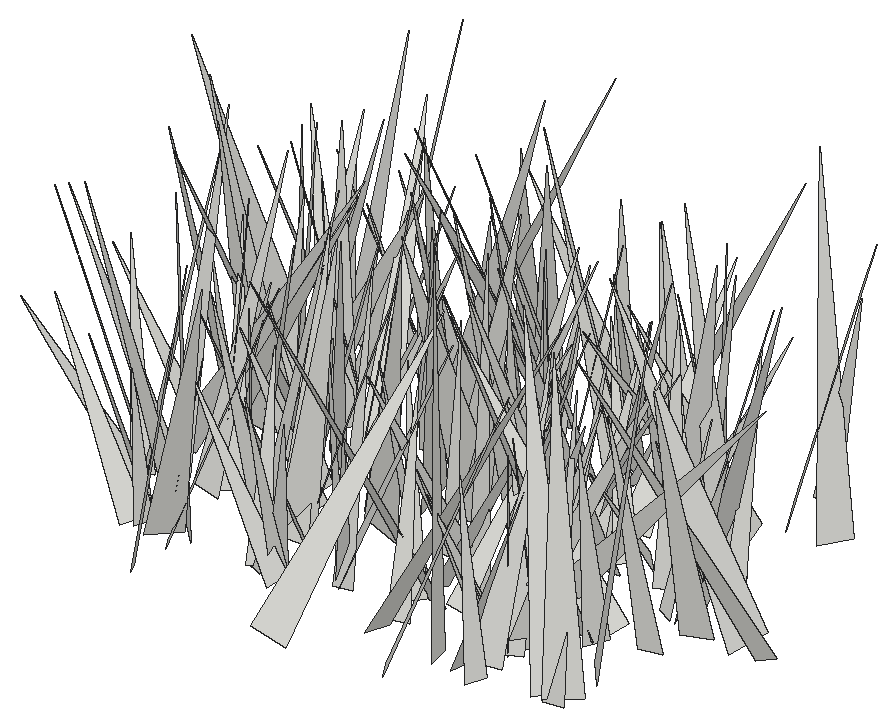
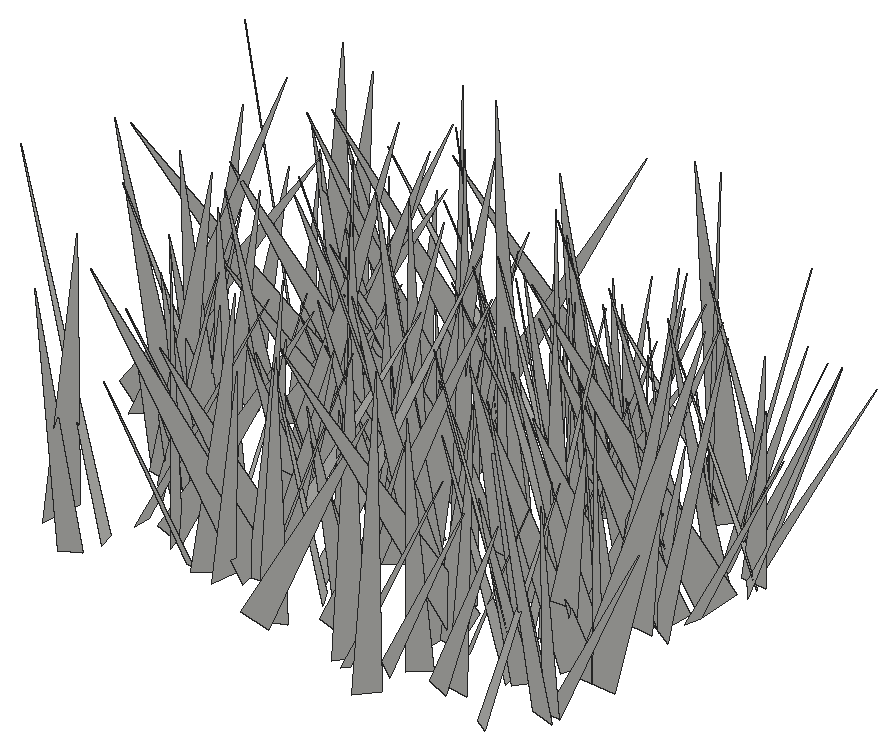
# SketchUp Ruby script. Lengths in inches.
U = 1.inch
M = Sketchup.active_model
def pt(a) = Geom::Point3d.new(a.map { |v| v * U })
def face(e, loops, mat)
  f = e.add_face(loops[0].map { |a| pt(a) })
  loops[1..].each { |l| e.add_face(l.map { |a| pt(a) }).erase! }
  f.material = f.back_material = mat if mat
  f
end
# faces: each face lists its corners as indices into pts; further lists are holes
def faces(e, pts, list, mat = nil) = list.each { |f| face(e, (f[0].is_a?(Array) ? f : [f]).map { |l| l.map { |i| pts[i] } }, mat) }
# xy, xz, yz: faces in a plane at the given z, y or x. An outline is a flat list of corners, or four numbers for a rectangle; further outlines are holes
def ring(l) = l.size == 4 ? [[l[0], l[1]], [l[2], l[1]], [l[2], l[3]], [l[0], l[3]]] : l.each_slice(2).to_a
def flat(e, list, mat, &to3) = list.each { |f| face(e, (f[0].is_a?(Array) ? f : [f]).map { |l| ring(l).map { |u, v| to3.(u, v) } }, mat) }
def xy(e, z, list, mat = nil) = flat(e, list, mat) { |x, y| [x, y, z] }
def xz(e, y, list, mat = nil) = flat(e, list, mat) { |x, z| [x, y, z] }
def yz(e, x, list, mat = nil) = flat(e, list, mat) { |y, z| [x, y, z] }
def lines(e, pts, list) = list.each { |a, b| e.add_line(pt(pts[a]), pt(pts[b])) }
# prism: a flat outline (further loops are holes) pulled along v
def prism(e, loops, v, mat = nil)
  f = face(e, loops, mat); d = Geom::Vector3d.new(v.map { |x| x * U })
  f.pushpull(f.normal.samedirection?(d) ? d.length : -d.length)
end
def box(e, o, s, mat = nil) = prism(e, [[o, [o[0] + s[0], o[1], o[2]], [o[0] + s[0], o[1] + s[1], o[2]], [o[0], o[1] + s[1], o[2]]]], [0, 0, s[2]], mat)
def at(x, y, z, deg = 0) = Geom::Transformation.translation(pt([x, y, z])) * Geom::Transformation.rotation(ORIGIN, Z_AXIS, deg.degrees)
def axes(o, x, y, z) = Geom::Transformation.new([*x, 0, *y, 0, *z, 0, *pt(o).to_a, 1])
def part(name) = M.definitions.add(name)
# library, detail: a bought-in or finely detailed component or shape, given as its bounding box
def library(name, o, s) = part(name).tap { |d| box(d.entities, o, s) }
def detail(e, o, s) = box(e.add_group.entities, o, s)
def put(e, d, t, mat = nil) = e.add_instance(d, t).tap { |i| i.material = mat if mat }
def group(e, t, mat = nil) = e.add_group.tap { |g| g.transformation = t; g.material = mat if mat }.entities
root = M.entities
c1 = part("fur_instance\#9")
p = [[0.8125,0,1.79],[0.67,-0.02,1.48],[0,-0.11,0],[0,0.11,0]]
faces(c1.entities,p,[[0,1,2,3]])
put(root,c1,axes([84.93,28.2,-27.1],[-3.91308,1.33626,1.31278],[1.41439,4.10109,0.04154],[1.2282,-0.46546,4.13474]))
put(root,c1,axes([68.6,29.75,-27.1],[5.57249,-4.36069,0.56036],[-4.38496,-5.5781,0.19774],[-0.31889,0.50141,7.07313]))
put(root,c1,axes([81.72,26.67,-27.1],[5.03516,3.5658,0.22039],[3.50469,-5.00395,0.89105],[-0.69327,0.6016,6.10523]))
put(root,c1,axes([76.67,25.97,-27.1],[-0.73588,7.38124,0.25307],[6.98236,0.77818,-2.39362],[2.40696,-0.00075,7.02103]))
put(root,c1,axes([69.36,26.85,-27.1],[4.53649,3.63122,1.57008],[3.09166,-4.74451,2.04009],[-2.46831,0.73111,5.44092]))
put(root,c1,axes([74.26,29.53,-27.1],[-4.45422,0.97791,0.2811],[1.01486,4.3608,0.91044],[0.07343,-0.95002,4.4685]))
put(root,c1,axes([73.88,30.16,-27.1],[-3.9744,-0.24759,1.6573],[0.13335,4.20562,0.94807],[1.67038,-0.92483,3.8676]))
put(root,c1,axes([67.49,29.9,-27.1],[2.92591,-1.89098,1.19539],[-1.88086,-3.14489,-0.37117],[-1.21125,0.31559,3.46396]))
put(root,c1,axes([73.47,30.54,-27.1],[0.57309,-4.07864,0.58369],[-4.03575,-0.43699,0.90892],[0.82985,0.69149,4.01716]))
put(root,c1,axes([67.57,30.38,-27.1],[-2.05359,-3.75931,0.63579],[-3.81243,2.01617,-0.39286],[-0.04503,0.74602,4.26559]))
put(root,c1,axes([88.39,29.16,-27.1],[-4.52139,5.22079,2.42729],[5.56937,4.74843,0.161],[1.45961,-1.94607,6.90462]))
put(root,c1,axes([67.04,29.79,-27.1],[-3.88022,2.75048,0.41463],[2.75578,3.70465,1.21426],[-0.37781,-1.22622,4.59857]))
put(root,c1,axes([69.24,30.39,-27.1],[-4.9247,-5.05159,2.9073],[-5.39927,5.38751,0.21521],[2.19519,1.91829,7.05159]))
put(root,c1,axes([80.1,31.94,-27.1],[-3.80092,-6.72254,0.0507],[-6.48684,3.65215,-2.05545],[-1.76524,1.05421,7.4441]))
put(root,c1,axes([82.68,28.74,-27.1],[-7.45834,-2.27512,2.73301],[-2.96816,7.48025,-1.87304],[1.95846,2.67246,7.56933]))
put(root,c1,axes([84.33,30.9375,-27.1],[-3.42009,-2.62307,1.97794],[-2.56254,3.91671,0.76324],[2.05575,0.51835,4.24205]))
put(root,c1,axes([87.82,29.27,-27.1],[-6.04844,4.67756,1.28768],[4.75602,6.12308,0.0974],[0.95811,-0.86582,7.6455]))
put(root,c1,axes([75.96,31.41,-27.1],[3.91592,-0.46866,0.80636],[-0.26131,-3.89224,-0.99321],[-0.89531,-0.91384,3.81675]))
put(root,c1,axes([84.44,29.37,-27.1],[-2.07384,5.25709,1.74566],[5.26815,2.4479,-1.11335],[1.712,-1.16445,5.54061]))
put(root,c1,axes([88.37,28.6,-27.1],[1.19098,5.93826,0.851],[5.76454,-1.37303,1.51343],[-1.66049,-0.50738,5.86438]))
put(root,c1,axes([82.39,32.1,-27.1],[-3.37943,-0.96857,0.84627],[-0.6019,3.29348,1.36586],[1.13667,-1.13567,3.23931]))
put(root,c1,axes([73,29.98,-27.1],[-1.62337,4.08317,1.17277],[4.21606,1.70273,-0.09236],[0.52201,-1.05424,4.39307]))
put(root,c1,axes([82.14,32.07,-27.1],[0.37183,-3.94608,0.38846],[-3.8933,-0.43727,-0.71534],[-0.75144,0.31297,3.89847]))
put(root,c1,axes([65.42,32.36,-27.1],[-4.70731,-0.314,0.0439],[-0.28456,4.4722,1.47573],[0.13983,-1.46975,4.48103]))
put(root,c1,axes([79.5,29.03,-27.1],[7.73901,0.54751,0.09462],[0.50511,-7.48314,1.98706],[-0.23147,1.9758,7.49957]))
put(root,c1,axes([83.77,28.63,-27.1],[6.82922,2.21825,1.16198],[1.82522,-6.72015,2.10172],[-1.71447,1.68168,6.86597]))
put(root,c1,axes([79.75,29.98,-27.1],[-0.43977,4.5707,0.64422],[4.59918,0.3789,0.45132],[-0.39225,-0.6818,4.56957]))
put(root,c1,axes([69.25,29.11,-27.1],[4.51704,3.2359,0.24642],[3.07452,-4.40221,1.45028],[-1.0388,1.04161,5.3639]))
put(root,c1,axes([66.73,32.49,-27.1],[-6.28754,-2.52373,1.27093],[-2.51372,6.41179,0.29625],[1.29062,0.19325,6.76865]))
put(root,c1,axes([75.96,31.16,-27.1],[4.98455,3.49636,0.32674],[3.50629,-4.92427,-0.79656],[0.19289,-0.83908,6.03621]))
put(root,c1,axes([88.13,31.47,-27.1],[5.88152,4.86813,2.28116],[5.13014,-6.09312,-0.22398],[-1.60749,-1.63397,7.63157]))
put(root,c1,axes([71.04,32.7,-27.1],[-4.89796,-0.50596,1.28828],[-0.38248,5.0478,0.52832],[1.33018,-0.4116,4.8956]))
put(root,c1,axes([66.65,32.99,-27.1],[3.46775,1.51161,0.84573],[1.722,-3.21287,-1.3182],[-0.18693,-1.55498,3.54578]))
put(root,c1,axes([72.72,32.56,-27.1],[2.84119,-6.18581,2.36185],[-6.62137,-2.65127,1.02137],[0.00779,2.57322,6.73004]))
put(root,c1,axes([75.22,32.19,-27.1],[1.82668,3.73793,1.95155],[3.99067,-2.21946,0.51574],[-1.36206,-1.48974,4.1283]))
put(root,c1,axes([84.125,32.78,-27.1],[-3.08736,-2.6391,1.38175],[-2.74426,3.29386,0.15946],[1.15895,0.7691,4.05847]))
put(root,c1,axes([72.91,29.76,-27.1],[4.10406,6.33899,0.98584],[6.11766,-4.2195,1.66374],[-1.93105,0.10466,7.36601]))
put(root,c1,axes([73.32,32.36,-27.1],[-3.16767,-3.69393,0.44061],[-3.42422,2.66901,-2.24153],[-1.45395,1.76199,4.31912]))
put(root,c1,axes([86.07,33.41,-27.1],[-4.08084,-6.31933,0.93728],[-6.28934,3.77891,-1.90517],[-1.12095,1.80323,7.27719]))
put(root,c1,axes([78.36,33.12,-27.1],[-4.55771,-1.35516,1.4154],[-1.26006,4.77117,0.51063],[1.50069,-0.10962,4.72742]))
put(root,c1,axes([79.8125,34.55,-27.1],[1.26749,-5.25605,0.55346],[-5.00773,-1.37633,-1.60227],[-1.68968,0.13629,5.16385]))
put(root,c1,axes([84.64,31.13,-27.1],[4.97283,-0.90694,1.68915],[-1.45035,-4.85051,1.66547],[-1.25389,2.01364,4.77261]))
put(root,c1,axes([86.66,33.32,-27.1],[3.6689,-2.8215,1.45683],[-2.81207,-3.92099,-0.512],[-1.47496,0.45716,4.59995]))
put(root,c1,axes([78.65,31.16,-27.1],[5.2038,5.70361,2.35891],[5.67233,-5.63566,1.11317],[-2.43315,-0.93989,7.64013]))
put(root,c1,axes([82.17,34.89,-27.1],[1.01842,-6.5564,0.3467],[-5.92672,-0.76709,2.90332],[2.82498,0.75429,5.9661]))
put(root,c1,axes([74.91,35,-27.1],[-0.13317,-8.12567,1.45261],[-7.87911,0.55826,2.40046],[2.46092,1.34765,7.76415]))
put(root,c1,axes([76.51,30.67,-27.1],[1.43264,6.02249,0.66756],[5.77311,-1.565,1.72927],[-1.84042,-0.22107,5.94411]))
put(root,c1,axes([79.24,31.66,-27.1],[-4.35702,1.54483,0.37411],[1.45493,4.3157,-0.87633],[0.64002,0.7059,4.53896]))
put(root,c1,axes([84.7,30.58,-27.1],[-5.37291,2.30629,0.61766],[1.96946,5.14098,-2.06404],[1.34972,1.6793,5.47055]))
put(root,c1,axes([65.08,33.22,-27.1],[-4.61833,-3.74237,0.73758],[-3.79853,4.40694,-1.4242],[-0.34716,1.56584,5.77113]))
put(root,c1,axes([84.61,33.04,-27.1],[2.40837,2.51325,1.53163],[2.71206,-2.66382,0.10655],[-1.14326,-1.0248,3.47927]))
put(root,c1,axes([72.71,32.33,-27.1],[-0.45657,6.34549,1.8425],[6.59681,0.54314,-0.23589],[0.37708,-1.81886,6.35752]))
put(root,c1,axes([66.14,33.47,-27.1],[-6.00367,-1.40851,0.07652],[-1.40991,5.98159,-0.51624],[-0.04369,0.52005,6.14503]))
put(root,c1,axes([71.98,34.82,-27.1],[-4.35378,0.44066,1.23045],[0.84047,4.2213,1.46212],[1.0009,-1.62788,4.12453]))
put(root,c1,axes([69.75,33.64,-27.1],[3.22406,2.21993,1.84513],[2.48282,-3.54361,-0.0749],[-1.47248,-1.11442,3.91371]))
put(root,c1,axes([88.67,34.09,-27.1],[-0.10037,-5.00985,1.67679],[-5.24561,-0.10471,-0.62683],[-0.62754,1.67652,4.9715]))
put(root,c1,axes([86.66,34.27,-27.1],[-6.39943,2.86094,0.01202],[2.71801,6.07041,2.2137],[-0.89308,-2.0256,6.65111]))
put(root,c1,axes([83.79,31.79,-27.1],[5.89458,-2.32049,1.52507],[-2.76984,-5.16651,2.8446],[-0.1962,3.22166,5.6603]))
put(root,c1,axes([65.08,32.84,-27.1],[-0.91318,4.58049,0.90258],[4.61205,0.74242,0.89849],[-0.72428,-1.04754,4.5834]))
put(root,c1,axes([80.95,32.06,-27.1],[-0.63847,4.33122,0.11328],[4.14955,0.64421,-1.24344],[1.2464,0.07394,4.19773]))
put(root,c1,axes([83.72,32.78,-27.1],[6.0984,-4.54505,0.22334],[-3.82324,-4.91501,4.37303],[2.46783,3.61705,6.22291]))
put(root,c1,axes([82.7,34.5,-27.1],[-2.40754,3.72637,1.88833],[4.14407,2.40561,0.53634],[0.52762,-1.89079,4.40391]))
put(root,c1,axes([79.36,32.97,-27.1],[5.44463,0.12063,0.24069],[0.04962,-5.23956,1.50366],[-0.26462,1.49964,5.23426]))
put(root,c1,axes([89.36,36.04,-27.1],[1.80262,-6.00522,1.15434],[-6.08405,-1.88243,-0.2921],[-0.61598,1.01901,6.26312]))
put(root,c1,axes([69.51,34.23,-27.1],[5.12051,1.66894,1.66295],[1.70709,-5.37015,0.13306],[-1.62376,-0.38277,5.38398]))
put(root,c1,axes([83.625,36.18,-27.1],[-0.04463,-6.97717,1.39975],[-6.92736,-0.27772,-1.60522],[-1.62845,1.37265,6.79015]))
put(root,c1,axes([80.7,33.66,-27.1],[1.55743,6.34801,1.89562],[6.44853,-1.89902,1.06134],[-1.51893,-1.55328,6.44953]))
put(root,c1,axes([69.49,35.1875,-27.1],[3.75751,0.05108,0.3502],[0.07903,-3.76142,-0.29936],[-0.34497,-0.30538,3.74592]))
put(root,c1,axes([65.375,32.4375,-27.1],[4.3588,4.87451,1.02077],[4.50794,-4.43827,1.9448],[-2.11691,0.58556,6.24322]))
put(root,c1,axes([92.48,36.36,-27.1],[-2.35699,-6.63901,0.53799],[-6.01099,1.87426,-3.2057],[-2.86948,1.52709,6.27339]))
put(root,c1,axes([67.8,33.28,-27.1],[1.8777,6.7714,0.98346],[6.8334,-1.90815,0.09124],[-0.35155,-0.923,7.02632]))
put(root,c1,axes([84.88,36.03,-27.1],[-2.69174,-3.80387,0.07847],[-3.66679,2.56798,-1.29661],[-1.01502,0.8106,4.47591]))
put(root,c1,axes([73.19,34.08,-27.1],[3.15484,4.86518,0.39731],[4.85003,-3.07066,-0.91053],[0.55227,-0.82578,5.72659]))
put(root,c1,axes([71.21,36.06,-27.1],[5.75664,2.23558,0.62086],[2.31995,-5.52205,-1.62697],[0.03364,-1.74108,5.95732]))
put(root,c1,axes([67.2,35.17,-27.1],[-4.37143,-2.8181,2.86453],[-3.24687,4.97094,-0.06453],[2.3675,1.61389,5.20067]))
put(root,c1,axes([83.4,34.28,-27.1],[1.4103,3.34023,0.25009],[3.32818,-1.428,0.30438],[-0.37801,-0.11091,3.61295]))
put(root,c1,axes([70.47,37.94,-27.1],[-2.5118,-6.70095,1.69222],[-6.07027,2.9998,2.86854],[3.30427,0.41708,6.55616]))
put(root,c1,axes([69.82,37.16,-27.1],[0.42063,-4.67833,0.35233],[-4.37367,-0.26302,1.72907],[1.69763,0.48155,4.36738]))
put(root,c1,axes([91.18,36.89,-27.1],[-7.69272,2.37823,1.5322],[2.71051,7.46743,2.01798],[0.8104,-2.40066,7.79498]))
put(root,c1,axes([83.34,37.9375,-27.1],[-0.92127,-7.60318,0.93237],[-7.64439,0.85236,-0.60268],[-0.49091,0.99576,7.63504]))
put(root,c1,axes([71.22,36.24,-27.1],[-4.01235,0.08097,0.58825],[0.14386,4.03101,0.42638],[0.5761,-0.44265,3.99045]))
put(root,c1,axes([66.02,33.77,-27.1],[1.84085,7.01016,1.12106],[6.97031,-2.00445,1.08846],[-1.34679,-0.79226,7.16563]))
put(root,c1,axes([78.15,35.08,-27.1],[0.81104,4.54834,1.26147],[4.65262,-0.98593,0.56355],[-0.7949,-1.13006,4.58559]))
put(root,c1,axes([82.19,36.17,-27.1],[3.78368,4.97369,3.03573],[5.56614,-4.15585,-0.12867],[-1.72376,-2.50217,6.24798]))
put(root,c1,axes([68.58,33.97,-27.1],[-4.8792,2.06982,0.10093],[1.96371,4.70056,-1.46614],[0.66196,1.31208,5.09325]))
put(root,c1,axes([73.58,36.33,-27.1],[4.19942,-1.36084,1.21546],[-1.38514,-4.36301,-0.09922],[-1.1877,0.2767,4.41329]))
put(root,c1,axes([65.04,36.6,-27.1],[-4.32306,0.06447,0.02072],[0.06687,4.27292,0.65655],[0.01068,-0.65679,4.2734]))
put(root,c1,axes([74.94,38.18,-27.1],[7.73874,0.04549,1.82687],[0.5794,-7.60007,-2.26513],[-1.73315,-2.33761,7.39995]))
put(root,c1,axes([82.67,34.16,-27.1],[5.53562,0.75174,0.06867],[0.66774,-5.11345,2.14935],[-0.35205,2.12143,5.1564]))
put(root,c1,axes([75.98,39.46,-27.1],[6.63906,-4.24471,1.17982],[-3.75911,-6.57064,-2.48644],[-2.29753,-1.51516,7.47745]))
put(root,c1,axes([65.96,36.84,-27.1],[1.53162,3.70831,1.75315],[4.01532,-0.97314,-1.44953],[0.83802,-2.1148,3.74116]))
put(root,c1,axes([67.28,35.95,-27.1],[0.68239,3.8164,1.4602],[3.78451,-1.14857,1.23331],[-1.54098,-1.13076,3.67553]))
put(root,c1,axes([64.98,35.11,-27.1],[6.90826,-2.9112,0.5406],[-2.88435,-6.30625,2.89882],[0.66922,2.87186,6.91346]))
put(root,c1,axes([82.61,35,-27.1],[-6.55431,0.09701,1.7896],[-0.34688,6.588,-1.62754],[1.75834,1.66126,6.34976]))
put(root,c1,axes([88,38.43,-27.1],[-4.12038,-2.11418,1.50488],[-1.47976,4.23386,1.89649],[2.13184,-1.14743,4.225]))
put(root,c1,axes([71.97,35.79,-27.1],[3.98122,4.30027,2.75674],[4.211,-4.74141,1.31475],[-2.89126,-0.98426,5.71085]))
put(root,c1,axes([77.15,37.69,-27.1],[2.1882,-4.93746,0.79161],[-4.93819,-1.99768,1.19031],[0.78701,1.19336,5.26781]))
put(root,c1,axes([80.67,36.34,-27.1],[-3.32037,-5.8988,2.51801],[-6.36421,2.67847,-2.11746],[-0.7956,3.19234,6.42939]))
put(root,c1,axes([66.33,38.34,-27.1],[-0.95753,-7.17721,1.84222],[-7.39469,1.0444,0.22542],[0.47406,1.79439,7.23729]))
put(root,c1,axes([84.38,39.55,-27.1],[-2.58943,-3.13022,0.07236],[-2.65217,2.2427,2.10831],[1.66419,-1.2964,3.47253]))
put(root,c1,axes([73.65,34.55,-27.1],[5.66789,4.81372,1.80284],[4.22946,-5.89252,2.43659],[-2.92126,0.80836,7.02566]))
put(root,c1,axes([68.09,39,-27.1],[-3.16334,-6.14078,0.476],[-6.132,3.08971,-0.89149],[-0.57823,0.82883,6.8499]))
put(root,c1,axes([87.19,38.09,-27.1],[2.31724,-3.70248,0.25487],[-3.62607,-2.19471,1.08527],[0.79054,0.78602,4.23086]))
put(root,c1,axes([65.41,38.1,-27.1],[-3.32824,-5.52708,1.61735],[-5.74671,3.30884,-0.51825],[0.37393,1.65668,6.43096]))
put(root,c1,axes([87.33,36.66,-27.1],[1.79566,3.71313,0.76849],[3.77743,-1.82574,-0.00496],[-0.33004,-0.69403,4.12452]))
put(root,c1,axes([77.35,37.58,-27.1],[5.13352,5.29295,1.04527],[5.31008,-4.70157,-2.27141],[0.95446,-2.31104,7.01492]))
put(root,c1,axes([68.92,38.95,-27.1],[5.69332,3.04756,1.30745],[3.31373,-5.12843,-2.47574],[0.12746,-2.79687,5.96424]))
put(root,c1,axes([65.43,37.1875,-27.1],[6.30652,-2.10429,0.15189],[-2.07978,-6.12031,1.56194],[0.35446,1.52876,6.46224]))
put(root,c1,axes([76.74,38.55,-27.1],[1.64053,-3.56149,0.70323],[-3.59089,-1.47867,0.88831],[0.53314,0.99969,3.81922]))
put(root,c1,axes([66.89,39.04,-27.1],[6.73753,-0.02978,4.19134],[0.53715,-7.86314,-0.91932],[-4.15689,-1.06433,6.67458]))
put(root,c1,axes([78.25,38.93,-27.1],[4.81176,-1.3762,1.70282],[-1.26945,-5.10354,-0.53746],[-1.78382,-0.0803,4.97575]))
put(root,c1,axes([86.23,38.3,-27.1],[-2.39493,4.93051,2.15105],[5.27679,2.61079,-0.10925],[1.04521,-1.88321,5.4803]))
put(root,c1,axes([87.83,36.74,-27.1],[5.27233,3.79468,0.9806],[3.62511,-5.34626,1.19781],[-1.48988,0.42019,6.38454]))
put(root,c1,axes([75.34,39.72,-27.1],[0.9927,-7.18833,2.00129],[-7.23058,-0.4281,2.04891],[1.84279,2.19257,6.96128]))
put(root,c1,axes([76.23,38.21,-27.1],[4.34648,-1.55951,0.20323],[-1.53377,-4.07129,1.56122],[0.34774,1.53551,4.34586]))
put(root,c1,axes([84.6,40.9,-27.1],[0.33482,-6.22736,0.74708],[-6.26175,-0.28913,0.39628],[0.3585,0.76592,6.22375]))
put(root,c1,axes([81.875,39.625,-27.1],[6.64605,0.23955,0.93352],[0.28653,-6.70181,-0.32012],[-0.92019,-0.35664,6.64266]))
put(root,c1,axes([72.625,40.93,-27.1],[0.91835,-4.65892,0.5996],[-4.68613,-0.86646,0.44487],[0.32448,0.67241,4.72768]))
put(root,c1,axes([69.25,41.23,-27.1],[-4.71687,-4.84842,1.35584],[-4.8132,4.8877,0.73342],[1.47602,0.44449,6.72444]))
put(root,c1,axes([86.52,40.44,-27.1],[7.28234,-1.08518,0.65082],[-1.04869,-7.30325,-0.44316],[-0.70811,-0.34428,7.3494]))
put(root,c1,axes([82.45,38.16,-27.1],[-3.28423,2.60896,0.74342],[2.31234,3.30268,-1.37511],[1.4186,0.65664,3.96257]))
put(root,c1,axes([83.69,38.85,-27.1],[-4.1604,2.35856,0.20079],[2.33408,4.15517,-0.44576],[0.39395,0.28953,4.76162]))
put(root,c1,axes([85.84,39.73,-27.1],[-2.17723,3.86998,1.04919],[4.00343,2.16477,0.32287],[0.22393,-1.07466,4.42864]))
put(root,c1,axes([68.23,40.75,-27.1],[-4.38219,4.14776,3.28171],[4.71988,4.98997,-0.0042],[2.38668,-2.25242,6.03386]))
put(root,c1,axes([82.37,38.66,-27.1],[-4.0426,1.99311,1.15136],[1.52694,4.06338,-1.67276],[1.72237,1.07573,4.18533]))
put(root,c1,axes([81.2,38.59,-27.1],[1.74005,3.73475,0.21366],[3.48509,-1.70407,1.40429],[-1.35946,0.41179,3.87351]))
put(root,c1,axes([68.85,37.13,-27.1],[-5.84983,3.65343,0.11485],[3.32744,5.4123,-2.68634],[1.51292,2.22277,6.35229]))
put(root,c1,axes([84.25,41.6875,-27.1],[4.71855,-5.46855,1.25045],[-5.59838,-4.69426,0.59612],[-0.35606,1.33873,7.19821]))
put(root,c1,axes([70,40.8125,-27.1],[4.56637,-2.19972,0.30987],[-2.21681,-4.46657,0.96025],[0.14341,0.99877,4.97679]))
put(root,c1,axes([65.95,40.28,-27.1],[0.08928,4.21713,1.27448],[4.4055,-0.088,-0.01741],[-0.00879,-1.27457,4.21804]))
put(root,c1,axes([76.69,40.25,-27.1],[-0.20342,5.45726,1.92359],[5.57072,0.70526,-1.41173],[1.56492,-1.80117,5.27542]))
put(root,c1,axes([87.33,40.52,-27.1],[-0.80473,7.1427,2.6366],[7.51279,0.31449,1.44102],[-1.23607,-2.73867,7.04196]))
put(root,c1,axes([66.2,40.77,-27.1],[3.99026,4.07334,2.14881],[4.32029,-4.29562,0.12027],[-1.59518,-1.44473,5.70086]))
put(root,c1,axes([64.88,42.76,-27.1],[1.74253,-7.39949,2.19817],[-7.33714,-2.28781,-1.88496],[-2.39807,1.62304,7.36449]))
put(root,c1,axes([79.17,40.08,-27.1],[-0.87591,3.86506,0.33078],[3.84564,0.82067,0.59405],[-0.50909,-0.4507,3.91829]))
put(root,c1,axes([68.9,40.4,-27.1],[-3.88558,0.60859,0.85055],[0.43871,3.91906,-0.80001],[0.9494,0.67978,3.85072]))
put(root,c1,axes([78.1,42.91,-27.1],[-5.60021,-5.8066,0.30959],[-5.79691,5.54128,-0.92996],[-0.45638,0.8674,8.01337]))
put(root,c1,axes([86.94,41.48,-27.1],[-4.01127,-3.66818,1.32519],[-3.89401,3.87381,-1.06408],[0.2199,1.68524,5.33044]))
put(root,c1,axes([81.21,40.9,-27.1],[-6.43148,-3.95381,0.27263],[-3.76371,5.93049,-2.78112],[-1.24153,2.50351,7.01869]))
put(root,c1,axes([84.63,43.76,-27.1],[0.43766,-5.35462,0.13989],[-4.92597,-0.45748,-2.09965],[-2.10387,-0.04276,4.94519]))
put(root,c1,axes([88.47,39.42,-27.1],[-4.48023,1.71415,0.10108],[1.53614,4.12726,-1.90446],[0.76734,1.74596,4.4027]))
put(root,c1,axes([83.72,41.18,-27.1],[2.80072,3.68056,0.20092],[3.50306,-2.57922,-1.58339],[1.14693,-1.10998,4.34551]))
put(root,c1,axes([66.41,40.96,-27.1],[6.19902,-0.22924,1.58295],[-0.50577,-6.29178,1.06951],[-1.51739,1.16065,6.11037]))
put(root,c1,axes([66.17,42.14,-27.1],[4.35594,-4.3452,0.48537],[-4.22774,-4.01128,2.03138],[1.11472,1.7662,5.80763]))
put(root,c1,axes([71.08,39.52,-27.1],[-3.48559,6.14429,0.41822],[6.11379,3.5101,-0.61419],[0.74073,-0.05879,7.03735]))
put(root,c1,axes([71.57,43.6875,-27.1],[-1.87294,-5.65903,1.00828],[-5.62978,2.02003,0.87988],[1.16052,0.66634,5.89562]))
put(root,c1,axes([65.23,42.15,-27.1],[-4.85936,-1.80324,2.4582],[-1.94231,5.39639,0.11902],[2.34986,0.73149,5.18178]))
put(root,c1,axes([76.25,42.39,-27.1],[-3.7574,-4.18768,1.74578],[-4.4509,3.84178,-0.36412],[0.87968,1.55129,5.61445]))
put(root,c1,axes([86.07,43.66,-27.1],[-5.4104,-1.19331,0.05848],[-1.15989,5.3113,1.06983],[0.28647,-1.03242,5.43616]))
put(root,c1,axes([85.44,41.19,-27.1],[5.18015,0.30458,2.40247],[-0.20645,-5.59667,1.15468],[-2.41288,1.13276,5.059]))
put(root,c1,axes([67.82,41.3,-27.1],[-2.82943,5.24506,0.49337],[5.22615,2.72388,1.01368],[-0.66438,-0.91081,5.87271]))
put(root,c1,axes([79.9,44.38,-27.1],[-1.23587,-5.65616,0.92472],[-5.5483,1.41785,1.25724],[1.43652,0.61007,5.65145]))
put(root,c1,axes([75.2,45.61,-27.1],[-0.88458,-7.33954,0.10795],[-7.20369,0.84713,-1.43254],[-1.40973,0.27658,7.25253]))
put(root,c1,axes([67.17,43.61,-27.1],[1.41484,-4.55258,1.06253],[-4.54528,-1.07998,1.42506],[1.09333,1.40157,4.54939]))
put(root,c1,axes([77.49,41.67,-27.1],[3.33394,1.47543,1.26624],[0.9738,-3.44268,1.44745],[-1.68284,0.93087,3.34618]))
put(root,c1,axes([79.76,43.4,-27.1],[0.51311,-4.91857,2.52241],[-5.22585,-1.25725,-1.38854],[-1.80151,2.24614,4.74633]))
put(root,c1,axes([82.46,40.9,-27.1],[-2.9389,4.8588,0.20427],[4.55933,2.83593,-1.85926],[1.6918,0.79774,5.36547]))
put(root,c1,axes([84.16,43.98,-27.1],[5.47086,1.91538,2.35531],[2.21322,-5.83902,-0.39241],[-2.07794,-1.17628,5.78316]))
put(root,c1,axes([69.95,44.18,-27.1],[-3.92921,-1.09616,0.24918],[-1.11465,3.91653,-0.34741],[0.14562,0.40197,4.06442]))
put(root,c1,axes([76.04,43.86,-27.1],[2.99214,-2.75371,1.44433],[-3.06357,-2.95389,0.71483],[-0.53251,1.52102,4.0031]))
put(root,c1,axes([71.57,43.35,-27.1],[7.18053,-1.42617,1.70446],[-1.71997,-7.21687,1.20732],[-1.40743,1.54336,7.22055]))
put(root,c1,axes([76.97,43.96,-27.1],[4.26525,2.34746,1.0733],[2.44325,-4.34035,-0.2164],[-0.83252,-0.71113,4.86375]))
put(root,c1,axes([67.61,44.36,-27.1],[4.85217,1.44436,0.49792],[1.4914,-4.83766,-0.50049],[-0.33141,-0.62336,5.03778]))
put(root,c1,axes([81.73,45.11,-27.1],[3.82096,-4.05561,2.24215],[-4.19487,-4.26194,-0.56033],[-1.96935,1.20949,5.5438]))
put(root,c1,axes([80.11,43.37,-27.1],[-6.83624,-2.0461,0.45627],[-2.08301,6.45462,-2.26447],[-0.23611,2.29788,6.76704]))
put(root,c1,axes([67.02,44.4,-27.1],[2.18192,-3.03993,1.35648],[-3.32882,-1.9865,0.90262],[0.01238,1.6293,3.63142]))
put(root,c1,axes([86.24,45.6,-27.1],[7.20484,3.15988,1.15153],[3.35999,-6.88107,-2.14053],[-0.14588,-2.42624,7.57051]))
put(root,c1,axes([70.7,46.04,-27.1],[2.83156,-3.99697,0.33188],[-4.00855,-2.80696,0.39506],[0.13188,0.49882,4.88236]))
put(root,c1,axes([64.76,45.22,-27.1],[-2.53868,-3.44184,0.53172],[-3.38696,2.28677,-1.36858],[-0.81085,1.22404,4.05193]))
put(root,c1,axes([67.97,43.46,-27.1],[5.71474,5.0925,1.62445],[5.00095,-5.93344,1.00766],[-1.88756,-0.30227,7.58791]))
put(root,c1,axes([74.44,46.16,-27.1],[-1.9055,-4.08481,0.78377],[-4.15591,1.83492,-0.5407],[-0.16841,0.93717,4.47485]))
put(root,c1,axes([68.62,46.4,-27.1],[-1.39495,-5.41554,1.57218],[-5.52882,1.63221,0.71678],[1.10996,1.3242,5.54619]))
put(root,c1,axes([64.71,45.6,-27.1],[-0.60793,-4.00143,1.69165],[-4.28266,0.83877,0.44495],[0.72934,1.58988,4.02282]))
put(root,c1,axes([73.39,46.99,-27.1],[5.78336,-2.78291,1.02515],[-2.6557,-5.85961,-0.92463],[-1.32013,-0.40388,6.35113]))
put(root,c1,axes([82.56,45.13,-27.1],[2.24479,3.42751,0.35228],[3.3467,-2.06895,-1.19586],[0.81948,-0.93948,3.91878]))
put(root,c1,axes([80.94,45.1,-27.1],[-4.87312,1.26006,1.29377],[1.19613,5.04128,-0.40455],[1.35309,0.08157,5.01711]))
put(root,c1,axes([71.18,42.47,-27.1],[7.74445,1.42991,0.81828],[1.0012,-7.20795,3.11989],[-1.30836,2.94814,7.231]))
put(root,c1,axes([73.08,47.54,-27.1],[-3.99864,-1.03805,0.42764],[-0.78188,3.71014,1.695],[0.80565,-1.55139,3.76744]))
put(root,c1,axes([80.3,43.93,-27.1],[7.35163,-0.33714,0.71191],[-0.54127,-7.01692,2.26646],[-0.57229,2.30568,7.00167]))
put(root,c1,axes([66.24,47.88,-27.1],[-3.01664,-4.03882,0.35129],[-3.9528,3.02747,0.86334],[0.90049,-0.2406,4.96657]))
put(root,c1,axes([77.39,46.6,-27.1],[1.77747,-4.94769,1.74658],[-5.22789,-1.82695,0.145],[-0.44649,1.69476,5.25529]))
put(root,c1,axes([71.75,46.78,-27.1],[-2.18116,-3.44946,0.52539],[-3.41914,1.9894,-1.13316],[-0.6959,1.0372,3.92074]))
put(root,c1,axes([64.84,45.96,-27.1],[2.76981,6.05425,2.08045],[6.39697,-2.70498,-0.64491],[-0.24704,-2.16406,6.62646]))
put(root,c1,axes([69.35,46.64,-27.1],[-0.15517,3.72025,1.9318],[3.94772,-0.52047,1.31942],[-1.40985,-1.86683,3.48188]))
put(root,c1,axes([78.01,46.91,-27.1],[-2.55985,4.83206,1.74885],[4.89019,1.69025,2.4878],[-1.579,-2.59892,4.86955]))
put(root,c1,axes([88.86,45.06,-27.1],[-7.32985,2.37013,1.25415],[2.21242,7.40801,-1.06942],[1.51512,0.64882,7.62892]))
put(root,c1,axes([86.77,47.11,-27.1],[0.64184,-5.02818,1.67754],[-5.1921,-0.25617,1.21871],[1.0672,1.77778,4.9203]))
put(root,c1,axes([71.19,48.63,-27.1],[5.82388,-2.11588,0.96568],[-1.89422,-5.82584,-1.34106],[-1.34958,-0.95373,6.04946]))
